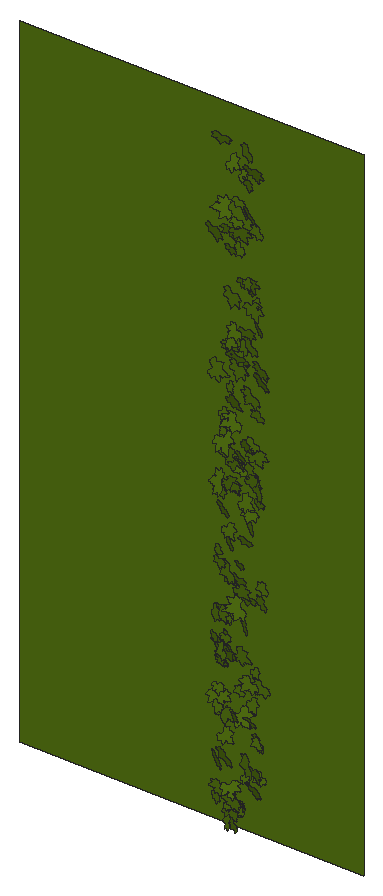
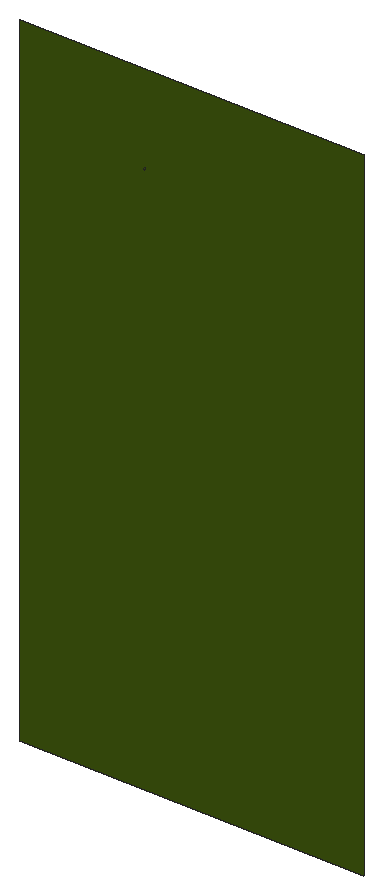
# SketchUp Ruby script. Lengths in inches.
U = 1.inch
M = Sketchup.active_model
def pt(a) = Geom::Point3d.new(a.map { |v| v * U })
def face(e, loops, mat)
  f = e.add_face(loops[0].map { |a| pt(a) })
  loops[1..].each { |l| e.add_face(l.map { |a| pt(a) }).erase! }
  f.material = f.back_material = mat if mat
  f
end
# faces: each face lists its corners as indices into pts; further lists are holes
def faces(e, pts, list, mat = nil) = list.each { |f| face(e, (f[0].is_a?(Array) ? f : [f]).map { |l| l.map { |i| pts[i] } }, mat) }
# xy, xz, yz: faces in a plane at the given z, y or x. An outline is a flat list of corners, or four numbers for a rectangle; further outlines are holes
def ring(l) = l.size == 4 ? [[l[0], l[1]], [l[2], l[1]], [l[2], l[3]], [l[0], l[3]]] : l.each_slice(2).to_a
def flat(e, list, mat, &to3) = list.each { |f| face(e, (f[0].is_a?(Array) ? f : [f]).map { |l| ring(l).map { |u, v| to3.(u, v) } }, mat) }
def xy(e, z, list, mat = nil) = flat(e, list, mat) { |x, y| [x, y, z] }
def xz(e, y, list, mat = nil) = flat(e, list, mat) { |x, z| [x, y, z] }
def yz(e, x, list, mat = nil) = flat(e, list, mat) { |y, z| [x, y, z] }
def lines(e, pts, list) = list.each { |a, b| e.add_line(pt(pts[a]), pt(pts[b])) }
# prism: a flat outline (further loops are holes) pulled along v
def prism(e, loops, v, mat = nil)
  f = face(e, loops, mat); d = Geom::Vector3d.new(v.map { |x| x * U })
  f.pushpull(f.normal.samedirection?(d) ? d.length : -d.length)
end
def box(e, o, s, mat = nil) = prism(e, [[o, [o[0] + s[0], o[1], o[2]], [o[0] + s[0], o[1] + s[1], o[2]], [o[0], o[1] + s[1], o[2]]]], [0, 0, s[2]], mat)
def at(x, y, z, deg = 0) = Geom::Transformation.translation(pt([x, y, z])) * Geom::Transformation.rotation(ORIGIN, Z_AXIS, deg.degrees)
def axes(o, x, y, z) = Geom::Transformation.new([*x, 0, *y, 0, *z, 0, *pt(o).to_a, 1])
def part(name) = M.definitions.add(name)
# library, detail: a bought-in or finely detailed component or shape, given as its bounding box
def library(name, o, s) = part(name).tap { |d| box(d.entities, o, s) }
def detail(e, o, s) = box(e.add_group.entities, o, s)
def put(e, d, t, mat = nil) = e.add_instance(d, t).tap { |i| i.material = mat if mat }
def group(e, t, mat = nil) = e.add_group.tap { |g| g.transformation = t; g.material = mat if mat }.entities
root = M.entities
M.materials.add("[Vegetation Blur 03]").color = [83, 114, 18]
c1 = part("ivy")
xy(c1.entities,0,[[0.782,0,0.786,0,0.787,0.005,0.789,0.009,0.821,0.072,0.875,0.147,1.001,0.272,1.073,0.331,1.137,0.363,1.178,0.379,1.223,0.384,1.272,0.383,1.311,0.374,1.36,0.355,1.399,0.334,1.491,0.285,1.541,0.244,1.583,0.199,1.617,0.15,1.64,0.128,1.662,0.115,1.717,0.105,1.745,0.093,1.784,0.054,1.819,0.057,1.854,0.064,1.882,0.075,1.896,0.074,1.91,0.071,1.937,0.063,1.964,0.053,1.99,0.038,2.016,0.015,2.034,0.002,2.04,0,2.038,0.003,2.036,0.007,2.033,0.038,2.036,0.068,2.045,0.1,2.055,0.116,2.064,0.123,2.077,0.129,2.088,0.129,2.106,0.132,2.118,0.13,2.179,0.132,2.207,0.133,2.225,0.133,2.242,0.138,2.22,0.162,2.207,0.186,2.206,0.213,2.212,0.236,2.228,0.262,2.247,0.274,2.298,0.283,2.355,0.294,2.37,0.296,2.376,0.295,2.377,0.3,2.377,0.303,2.385,0.329,2.411,0.37,2.426,0.392,2.449,0.407,2.511,0.426,2.561,0.444,2.619,0.466,2.589,0.469,2.561,0.476,2.501,0.5,2.449,0.516,2.424,0.523,2.401,0.535,2.377,0.556,2.372,0.568,2.36,0.575,2.268,0.586,2.225,0.592,2.207,0.599,2.194,0.61,2.143,0.65,2.13,0.664,2.122,0.682,2.123,0.7,2.13,0.719,2.148,0.75,2.17,0.781,2.195,0.807,2.221,0.828,2.284,0.874,2.291,0.88,2.288,0.887,2.276,0.9,2.267,0.916,2.265,0.933,2.273,0.967,2.292,1.002,2.313,1.03,2.334,1.054,2.348,1.067,2.358,1.074,2.363,1.076,2.362,1.081,2.35,1.094,2.347,1.11,2.35,1.143,2.359,1.18,2.385,1.254,2.415,1.324,2.448,1.393,2.45,1.4,2.446,1.398,2.44,1.394,2.427,1.383,2.402,1.36,2.376,1.339,2.345,1.324,2.305,1.309,2.282,1.303,2.273,1.306,2.245,1.294,2.212,1.287,2.187,1.291,2.163,1.301,2.142,1.316,2.134,1.327,2.124,1.325,2.09,1.292,2.053,1.259,2.014,1.234,1.973,1.215,1.954,1.21,1.931,1.208,1.909,1.212,1.893,1.22,1.879,1.233,1.872,1.248,1.867,1.281,1.864,1.319,1.821,1.258,1.773,1.197,1.726,1.141,1.698,1.121,1.679,1.116,1.666,1.117,1.647,1.122,1.632,1.129,1.62,1.141,1.617,1.154,1.617,1.219,1.621,1.254,1.623,1.268,1.623,1.281,1.618,1.314,1.606,1.346,1.603,1.375,1.607,1.403,1.603,1.467,1.599,1.499,1.605,1.525,1.614,1.552,1.629,1.577,1.635,1.589,1.629,1.587,1.618,1.582,1.596,1.566,1.581,1.556,1.568,1.552,1.557,1.55,1.545,1.553,1.531,1.562,1.522,1.572,1.504,1.591,1.486,1.611,1.474,1.631,1.457,1.666,1.455,1.684,1.457,1.698,1.452,1.715,1.444,1.728,1.424,1.754,1.419,1.772,1.423,1.786,1.434,1.819,1.444,1.848,1.446,1.855,1.44,1.861,1.43,1.867,1.386,1.904,1.349,1.948,1.326,1.973,1.31,1.995,1.288,2.048,1.284,2.153,1.287,2.254,1.284,2.255,1.282,2.253,1.278,2.247,1.274,2.237,1.266,2.216,1.226,2.125,1.208,2.076,1.184,2.033,1.155,1.984,1.135,1.942,1.111,1.899,1.083,1.861,1.053,1.85,1.059,1.83,1.061,1.809,1.056,1.79,1.049,1.767,1.04,1.749,1.018,1.733,0.994,1.726,0.942,1.734,0.95,1.6875,0.944,1.645,0.932,1.608,0.911,1.585,0.881,1.58,0.854,1.582,0.828,1.588,0.785,1.618,0.773,1.625,0.775,1.614,0.779,1.598,0.796,1.502,0.818,1.402,0.861,1.283,0.882,1.224,0.894,1.174,0.892,1.148,0.886,1.123,0.881,1.107,0.872,1.099,0.849,1.094,0.818,1.092,0.789,1.098,0.762,1.107,0.753,1.113,0.721,1.139,0.698,1.163,0.678,1.194,0.665,1.224,0.628,1.28,0.612,1.312,0.606,1.327,0.606,1.314,0.599,1.282,0.594,1.267,0.581,1.256,0.544,1.245,0.512,1.244,0.473,1.249,0.444,1.256,0.382,1.288,0.339,1.306,0.324,1.316,0.317,1.324,0.309,1.326,0.27,1.314,0.227,1.313,0.185,1.3125,0.152,1.317,0.122,1.328,0.092,1.345,0.073,1.353,0.079,1.338,0.092,1.308,0.117,1.249,0.13,1.215,0.139,1.164,0.147,1.148,0.157,1.136,0.163,1.122,0.174,1.086,0.177,1.067,0.182,1.054,0.186,1.043,0.191,1.038,0.211,1.028,0.237,1.005,0.25,0.974,0.253,0.96,0.25,0.944,0.242,0.914,0.243,0.906,0.249,0.902,0.26,0.894,0.289,0.88,0.307,0.873,0.322,0.862,0.364,0.799,0.403,0.738,0.431,0.709,0.439,0.691,0.441,0.678,0.4375,0.66,0.428,0.645,0.394,0.623,0.303,0.594,0.255,0.581,0.214,0.577,0.179,0.573,0.173,0.568,0.175,0.561,0.167,0.55,0.141,0.523,0.113,0.503,0.077,0.49,0.045,0.486,0.026,0.485,0.019,0.486,0.011,0.483,0,0.471,0.014,0.467,0.044,0.455,0.058,0.447,0.07,0.438,0.097,0.411,0.125,0.394,0.158,0.377,0.174,0.366,0.182,0.359,0.185,0.361,0.242,0.331,0.253,0.316,0.258,0.303,0.262,0.283,0.274,0.278,0.308,0.274,0.341,0.252,0.366,0.226,0.366,0.222,0.37,0.22,0.38,0.221,0.395,0.221,0.425,0.216,0.45,0.207,0.465,0.192,0.473,0.178,0.484,0.15,0.489,0.116,0.483,0.089,0.468,0.058,0.45,0.035,0.435,0.018,0.429,0.011,0.434,0.012,0.438,0.014,0.469,0.019,0.542,0.016,0.581,0.015,0.612,0.027,0.68,0.055,0.696,0.057,0.712,0.052,0.73,0.045,0.741,0.036,0.766,0.014]])
xz(root,174.5,[[114.28,101,138.74,147]],"[Vegetation Blur 03]")
put(root,c1,axes([128.08,173.7,139.49],[0.6079,-0.24736,0.08777],[0.11732,0.08596,-0.50313],[-0.11068,-1.26744,-0.05125]),"[Vegetation Blur 03]")
put(root,c1,axes([128.47,173.7,113.51],[0.3306,-0.20851,0.08999],[0.10594,-0.063,-0.2822],[-0.10584,-0.71438,-0.00138]),"[Vegetation Blur 03]")
put(root,c1,axes([128.72,173.7,113.4],[0.54219,-0.07189,-0.27942],[-0.3337,0.21166,-0.43986],[-0.08416,-1.30245,-0.05606]),"[Vegetation Blur 03]")
put(root,c1,axes([128.59,173.7,145.41],[0.46012,0.08661,-0.09796],[-0.12471,0.12465,-0.37281],[0.02504,-0.97055,-0.05662]),"[Vegetation Blur 03]")
put(root,c1,axes([128.5625,173.7,104.16],[0.58678,0.063,-0.19417],[-0.23912,0.05083,-0.47872],[0.01906,-1.30195,-0.02809]),"[Vegetation Blur 03]")
put(root,c1,axes([128.51,173.7,103.27],[0.34382,-0.15266,0.07768],[0.0934,-0.03785,-0.28706],[-0.07642,-0.73315,-0.00136]),"[Vegetation Blur 03]")
put(root,c1,axes([128.07,173.7,109.53],[0.59488,0.11123,0.16598],[0.20655,-0.0688,-0.48585],[0.04022,-1.29188,0.04016]),"[Vegetation Blur 03]")
put(root,c1,axes([128.54,173.7,106.05],[0.51362,-0.33546,-0.11294],[-0.11227,0.20752,-0.43703],[-0.18199,-1.07476,-0.04914]),"[Vegetation Blur 03]")
put(root,c1,axes([129.11,173.7,112.17],[0.24584,0.04332,-0.24097],[-0.29547,0.08344,-0.19842],[-0.01781,-0.78621,-0.03434]),"[Vegetation Blur 03]")
put(root,c1,axes([129.45,173.7,124.09],[0.21833,-0.37386,-0.44692],[-0.55988,0.15366,-0.2024],[-0.13932,-1.20335,0.113]),"[Vegetation Blur 03]")
put(root,c1,axes([129.2,173.7,106.26],[0.33588,0.02262,-0.39753],[-0.47681,0.26549,-0.26596],[-0.10014,-1.18823,-0.067]),"[Vegetation Blur 03]")
put(root,c1,axes([128.25,173.7,129.59],[0.09221,0.01276,0.54145],[0.66339,-0.02223,-0.07517],[-0.00985,-1.37816,0.00623]),"[Vegetation Blur 03]")
put(root,c1,axes([128.54,173.7,123.17],[0.25,-0.03131,0.17773],[0.21716,-0.03407,-0.2044],[-0.02234,-0.68141,0.00205]),"[Vegetation Blur 03]")
put(root,c1,axes([128.51,173.7,114.53],[0.13511,-0.04438,0.35866],[0.42367,-0.24214,-0.11102],[-0.11873,-0.91459,0.01199]),"[Vegetation Blur 03]")
put(root,c1,axes([128.75,173.7,109.24],[0.37736,-0.14693,-0.03133],[-0.04655,-0.08489,-0.31089],[-0.06637,-0.77592,0.03994]),"[Vegetation Blur 03]")
put(root,c1,axes([128.58,173.7,110.22],[0.36114,-0.04689,0.10699],[0.12628,-0.12494,-0.29255],[-0.0419,-0.78067,0.04039]),"[Vegetation Blur 03]")
put(root,c1,axes([128.98,173.7,112.5625],[0.39633,-0.13888,-0.234],[-0.27566,0.17367,-0.32719],[-0.1038,-0.99151,-0.02453]),"[Vegetation Blur 03]")
put(root,c1,axes([128.73,173.7,118.66],[0.10493,-0.03643,0.24088],[0.29195,-0.08918,-0.08683],[-0.04677,-0.63839,-0.00162]),"[Vegetation Blur 03]")
put(root,c1,axes([128.5625,173.7,122.63],[0.3534,-0.02851,0.14206],[0.17452,0.03242,-0.28817],[-0.00545,-0.81,-0.01653]),"[Vegetation Blur 03]")
put(root,c1,axes([128.7,173.7,118.42],[0.40755,-0.11351,-0.00014],[0.00098,0.01751,-0.33557],[-0.05515,-0.83847,-0.00699]),"[Vegetation Blur 03]")
put(root,c1,axes([129.01,173.7,122.03],[0.4235,-0.13743,-0.21645],[-0.24668,0.24247,-0.3457],[-0.1181,-0.99928,-0.05411]),"[Vegetation Blur 03]")
put(root,c1,axes([128.78,173.7,111.86],[0.26031,-0.0805,0.12545],[0.1556,0.01165,-0.21388],[-0.03078,-0.62197,-0.02024]),"[Vegetation Blur 03]")
put(root,c1,axes([128.65,173.7,115.28],[0.41549,-0.08208,0.11963],[0.15106,0.12998,-0.33542],[-0.01613,-0.89729,-0.05953]),"[Vegetation Blur 03]")
put(root,c1,axes([129.3125,173.7,113.2],[0.33509,-0.2609,-0.26753],[-0.3303,0.08476,-0.28857],[-0.12012,-0.96089,0.04719]),"[Vegetation Blur 03]")
put(root,c1,axes([129.64,173.7,113.78],[0.07952,-0.02515,-0.25316],[-0.29832,0.17612,-0.06516],[-0.08589,-0.63499,-0.00805]),"[Vegetation Blur 03]")
put(root,c1,axes([129.88,173.7,141.66],[0.17867,-0.14742,-0.47769],[-0.58909,-0.10072,-0.14187],[0.02629,-1.25528,0.06748]),"[Vegetation Blur 03]")
put(root,c1,axes([130.06,173.7,125.72],[0.10377,0.02186,-0.53621],[-0.65451,0.12482,-0.08356],[-0.05827,-1.36305,-0.01625]),"[Vegetation Blur 03]")
put(root,c1,axes([129.85,173.7,114.94],[0.04974,-0.00028,-0.27725],[-0.32677,0.19308,-0.03908],[-0.09286,-0.67961,-0.01099]),"[Vegetation Blur 03]")
put(root,c1,axes([129.9375,173.7,115.46],[0.08632,-0.07212,-0.36138],[-0.4424,0.06914,-0.07256],[-0.03977,-0.92577,0.02273]),"[Vegetation Blur 03]")
put(root,c1,axes([129.62,173.7,118.4375],[0.39881,-0.16855,-0.40776],[-0.49292,0.16963,-0.33214],[-0.11562,-1.30452,0.00949]),"[Vegetation Blur 03]")
put(root,c1,axes([128.95,173.7,127.48],[0.21376,-0.00368,0.2636],[0.3197,-0.11113,-0.17293],[-0.04601,-0.78924,0.02312]),"[Vegetation Blur 03]")
put(root,c1,axes([129.32,173.7,127.12],[0.30532,-0.22387,-0.07925],[-0.10993,-0.04866,-0.26046],[-0.09582,-0.65751,0.04626]),"[Vegetation Blur 03]")
put(root,c1,axes([129.85,173.7,102.12],[0.10497,-0.16799,-0.28426],[-0.34085,0.17977,-0.10055],[-0.10859,-0.72666,0.04084]),"[Vegetation Blur 03]")
put(root,c1,axes([129.12,173.7,113.5625],[0.3425,-0.04443,0.04433],[0.05384,-0.01893,-0.28004],[-0.02276,-0.71335,0.00467]),"[Vegetation Blur 03]")
put(root,c1,axes([128.69,173.7,109.03],[0.66487,-0.12258,0.05657],[0.06821,-0.03171,-0.54475],[-0.06083,-1.37523,0.00752]),"[Vegetation Blur 03]")
put(root,c1,axes([129.74,173.7,119.85],[0.19183,-0.05588,-0.2698],[-0.31224,0.23474,-0.15552],[-0.11192,-0.75067,-0.02855]),"[Vegetation Blur 03]")
put(root,c1,axes([128.74,173.7,114.98],[0.40007,-0.13518,0.27607],[0.33165,-0.13835,-0.33079],[-0.0935,-1.06919,0.0079]),"[Vegetation Blur 03]")
put(root,c1,axes([128.82,173.7,106.75],[0.24435,0.09355,0.35761],[0.44053,-0.04867,-0.19849],[0.00137,-1.03125,0.04181]),"[Vegetation Blur 03]")
put(root,c1,axes([128.52,173.7,125.74],[0.49312,0.07516,0.37451],[0.45503,-0.28887,-0.38996],[-0.06962,-1.3557,0.10386]),"[Vegetation Blur 03]")
put(root,c1,axes([129.34,173.7,102.54],[0.09713,0.02395,0.23937],[0.28996,-0.10667,-0.07669],[-0.04564,-0.62678,0.0222]),"[Vegetation Blur 03]")
put(root,c1,axes([129.15,173.7,132.24],[0.48068,0.01776,0.03152],[0.03794,0.06838,-0.39147],[0.01124,-0.98997,-0.02647]),"[Vegetation Blur 03]")
put(root,c1,axes([129.13,173.7,102.32],[0.46585,0.02288,0.14137],[0.17091,0.11775,-0.37813],[0.0303,-1.01595,-0.04064]),"[Vegetation Blur 03]")
put(root,c1,axes([129.68,173.7,113.05],[0.36602,-0.17334,-0.17958],[-0.2031,0.19186,-0.30487],[-0.11941,-0.85763,-0.0319]),"[Vegetation Blur 03]")
put(root,c1,axes([129.08,173.7,139.67],[0.63593,0.00439,0.02808],[0.0337,0.19557,-0.51321],[0.00724,-1.29586,-0.07736]),"[Vegetation Blur 03]")
put(root,c1,axes([129.51,173.7,138.55],[0.37054,-0.08411,-0.02834],[-0.02969,0.09383,-0.30232],[-0.04467,-0.76008,-0.03419]),"[Vegetation Blur 03]")
put(root,c1,axes([129.06,173.7,103.84],[0.46596,0.12424,0.22352],[0.28037,-0.18097,-0.37349],[0.00652,-1.09739,0.0869]),"[Vegetation Blur 03]")
put(root,c1,axes([129.39,173.7,117.06],[0.25004,-0.05522,0.19659],[0.24228,0.07618,-0.20189],[0.00655,-0.71038,-0.03693]),"[Vegetation Blur 03]")
put(root,c1,axes([129.89,173.7,103.81],[0.43018,0.03461,-0.33433],[-0.40999,0.03807,-0.35076],[-0.00059,-1.2218,-0.0204]),"[Vegetation Blur 03]")
put(root,c1,axes([129.32,173.7,112.03],[0.13975,-0.17275,0.35559],[0.44281,0.11446,-0.10717],[0.0284,-0.9346,-0.07885]),"[Vegetation Blur 03]")
put(root,c1,axes([129.14,173.7,120.2],[0.35229,-0.00554,0.29733],[0.36145,-0.12544,-0.28562],[-0.04568,-1.0353,0.03302]),"[Vegetation Blur 03]")
put(root,c1,axes([130.07,173.7,128.11],[0.3559,-0.06669,-0.38571],[-0.47242,-0.14005,-0.28653],[0.03508,-1.20938,0.05445]),"[Vegetation Blur 03]")
put(root,c1,axes([129.41,173.7,103.72],[0.62299,-0.15418,-0.12642],[-0.15294,0.05244,-0.51207],[-0.07884,-1.31998,-0.00558]),"[Vegetation Blur 03]")
put(root,c1,axes([129.38,173.7,131.97],[0.08788,0.15958,0.41108],[0.50211,-0.20702,-0.05886],[-0.08717,-1.03158,0.0754]),"[Vegetation Blur 03]")
put(root,c1,axes([128.98,173.7,123.21],[0.49372,-0.08066,0.3359],[0.41334,0.06825,-0.4021],[-0.00879,-1.32093,-0.04129]),"[Vegetation Blur 03]")
put(root,c1,axes([129.875,173.7,102.14],[0.34936,-0.1754,-0.17065],[-0.20005,0.12722,-0.29335],[-0.10473,-0.82812,-0.00892]),"[Vegetation Blur 03]")
put(root,c1,axes([129.7,173.7,123.82],[0.46927,-0.11869,-0.14311],[-0.17217,0.07416,-0.3857],[-0.06659,-1.02821,-0.0113]),"[Vegetation Blur 03]")
put(root,c1,axes([129.56,173.7,129.45],[0.20111,-0.0492,0.23305],[0.27447,-0.17313,-0.16352],[-0.08231,-0.69755,0.02415]),"[Vegetation Blur 03]")
put(root,c1,axes([129.61,173.7,131.9375],[0.61818,0.02753,-0.20694],[-0.25253,0.20999,-0.49806],[-0.0265,-1.35881,-0.08116]),"[Vegetation Blur 03]")
put(root,c1,axes([129.48,173.7,143.34],[0.1221,0.15901,0.36769],[0.45566,-0.11863,-0.09271],[-0.03634,-0.95319,0.07288]),"[Vegetation Blur 03]")
put(root,c1,axes([129.77,173.7,103.77],[0.53938,-0.11783,-0.24861],[-0.28048,0.34993,-0.43141],[-0.13192,-1.22575,-0.09926]),"[Vegetation Blur 03]")
put(root,c1,axes([129.49,173.7,109.0625],[0.49941,-0.26714,0.04177],[0.06827,0.12648,-0.4165],[-0.1217,-1.02529,-0.06226]),"[Vegetation Blur 03]")
put(root,c1,axes([130.68,173.7,141.38],[0.10747,0.09693,-0.42949],[-0.50045,0.37307,-0.07017],[-0.16944,-1.0404,-0.06517]),"[Vegetation Blur 03]")
put(root,c1,axes([129.47,173.7,135.95],[0.66254,-0.24066,-0.04091],[-0.05165,-0.00895,-0.54898],[-0.11628,-1.36725,0.01079]),"[Vegetation Blur 03]")
put(root,c1,axes([130.08,173.7,133.8],[0.41213,-0.1677,-0.21359],[-0.27008,-0.08234,-0.33694],[-0.04682,-1.00125,0.06348]),"[Vegetation Blur 03]")
put(root,c1,axes([130.57,173.7,116.5],[0.32603,-0.13943,-0.47145],[-0.58131,-0.12239,-0.26207],[0.01889,-1.35947,0.07195]),"[Vegetation Blur 03]")
put(root,c1,axes([130.01,173.7,140.4],[0.32282,0.01218,-0.05233],[-0.06347,-0.05325,-0.26277],[0.01083,-0.67519,0.01978]),"[Vegetation Blur 03]")
put(root,c1,axes([129.6,173.7,124.54],[0.35919,-0.07581,0.24051],[0.29623,0.02355,-0.29351],[-0.02119,-0.9558,-0.02631]),"[Vegetation Blur 03]")
put(root,c1,axes([130.18,173.7,141.8],[0.32239,-0.01176,-0.10948],[-0.13423,-0.01041,-0.2631],[-0.00333,-0.71849,0.00561]),"[Vegetation Blur 03]")
put(root,c1,axes([130.7,173.7,103.01],[0.06839,0.01536,-0.24268],[-0.29667,-0.04173,-0.0561],[0.02144,-0.62648,-0.00221]),"[Vegetation Blur 03]")
put(root,c1,axes([130.6,173.7,110.71],[0.15181,-0.00524,-0.23084],[-0.28286,-0.00517,-0.12389],[0.00101,-0.66057,0.0028]),"[Vegetation Blur 03]")
put(root,c1,axes([129.49,173.7,128.62],[0.38193,-0.25872,0.35613],[0.44798,0.02235,-0.31745],[-0.07443,-1.19311,-0.08317]),"[Vegetation Blur 03]")
put(root,c1,axes([130.93,173.7,114.9],[0.06026,0.01776,-0.40154],[-0.46093,0.35917,-0.04358],[-0.17229,-0.95467,-0.02387]),"[Vegetation Blur 03]")
put(root,c1,axes([130.36,173.7,125.6],[0.28037,-0.06157,-0.15463],[-0.18018,0.15229,-0.22714],[-0.06579,-0.67947,-0.0369]),"[Vegetation Blur 03]")
put(root,c1,axes([129.96,173.7,117.7],[0.47998,-0.11829,-0.01678],[-0.01365,0.11877,-0.39191],[-0.0595,-0.98146,-0.0454]),"[Vegetation Blur 03]")
put(root,c1,axes([130.1875,173.7,118.55],[0.3065,-0.10801,0.00878],[0.01921,0.10156,-0.25024],[-0.05001,-0.62289,-0.04232]),"[Vegetation Blur 03]")
put(root,c1,axes([129.91,173.7,131.42],[0.63233,-0.20373,-0.05495],[-0.06893,-0.01048,-0.5222],[-0.0979,-1.30853,0.01274]),"[Vegetation Blur 03]")
put(root,c1,axes([129.64,173.7,139.53],[0.56255,-0.01811,0.20546],[0.25121,0.13405,-0.45628],[0.01862,-1.26114,-0.05145]),"[Vegetation Blur 03]")
put(root,c1,axes([130.77,173.7,124.98],[0.19807,-0.04882,-0.25327],[-0.31096,-0.06252,-0.16009],[0.01294,-0.755,0.02963]),"[Vegetation Blur 03]")
put(root,c1,axes([130.14,173.7,125.22],[0.42582,-0.25778,-0.01572],[0.00049,0.14225,-0.35818],[-0.12674,-0.86554,-0.05419]),"[Vegetation Blur 03]")
put(root,c1,axes([130.65,173.7,120.24],[0.26692,0.10027,-0.19485],[-0.24358,0.09015,-0.21495],[0.00657,-0.73139,-0.05321]),"[Vegetation Blur 03]")
put(root,c1,axes([130.39,173.7,139.04],[0.38208,-0.19358,-0.10183],[-0.13229,-0.03969,-0.31874],[-0.08317,-0.82615,0.03917]),"[Vegetation Blur 03]")
put(root,c1,axes([129.7,173.7,108.34],[0.39393,0.1891,0.39235],[0.48905,-0.10099,-0.3194],[0.01969,-1.27498,0.08349]),"[Vegetation Blur 03]")
put(root,c1,axes([130.13,173.7,130.7],[0.23197,-0.0436,0.29061],[0.3566,0.00644,-0.18945],[-0.00894,-0.8745,-0.01588]),"[Vegetation Blur 03]")
put(root,c1,axes([131.08,173.7,106.44],[0.28462,-0.17247,-0.45638],[-0.54186,0.28495,-0.24203],[-0.16158,-1.25936,0.00774]),"[Vegetation Blur 03]")
put(root,c1,axes([129.94,173.7,116.58],[0.39343,-0.07208,0.30532],[0.37571,0.06003,-0.32024],[-0.0052,-1.11557,-0.03696]),"[Vegetation Blur 03]")
put(root,c1,axes([130.43,173.7,142.95],[0.0888,0.09674,0.25308],[0.31076,-0.1168,-0.0656],[-0.0424,-0.6534,0.0492]),"[Vegetation Blur 03]")
put(root,c1,axes([130.86,173.7,132.92],[0.29115,-0.21346,-0.2217],[-0.27097,0.0878,-0.25032],[-0.10549,-0.81469,0.03111]),"[Vegetation Blur 03]")
put(root,c1,axes([131.38,173.7,125.1],[0.14596,0.116,-0.44941],[-0.55223,-0.05004,-0.12149],[0.03805,-1.17121,-0.03932]),"[Vegetation Blur 03]")
put(root,c1,axes([130.11,173.7,112.21],[0.18573,-0.07263,0.44986],[0.55141,-0.04477,-0.15278],[-0.03192,-1.19609,-0.0216]),"[Vegetation Blur 03]")
put(root,c1,axes([130.61,173.7,116.51],[0.38415,0.08832,-0.09325],[-0.11924,0.10565,-0.31143],[0.02608,-0.81794,-0.0503]),"[Vegetation Blur 03]")
put(root,c1,axes([130.87,173.7,141.38],[0.42548,-0.09437,-0.33716],[-0.38139,0.39508,-0.33797],[-0.16527,-1.15464,-0.08808]),"[Vegetation Blur 03]")
put(root,c1,axes([130.9375,173.7,145.45],[0.35368,-0.15187,-0.29343],[-0.34945,0.17479,-0.29479],[-0.11221,-1.02299,-0.00681]),"[Vegetation Blur 03]")
put(root,c1,axes([131.05,173.7,108.8],[0.21856,0.08137,-0.22546],[-0.27868,0.10188,-0.17416],[-0.01478,-0.71768,-0.05028]),"[Vegetation Blur 03]")
put(root,c1,axes([130.53,173.7,104.72],[0.17985,0.03398,0.21034],[0.25744,-0.07475,-0.14472],[-0.02044,-0.64238,0.02797]),"[Vegetation Blur 03]")
put(root,c1,axes([131.03,173.7,133.11],[0.38374,-0.03816,-0.34105],[-0.41282,0.15382,-0.31209],[-0.06752,-1.15732,-0.03024]),"[Vegetation Blur 03]")
put(root,c1,axes([131.4,173.7,121.25],[0.07886,-0.02245,-0.3122],[-0.36365,0.24601,-0.06396],[-0.11923,-0.76517,-0.0114]),"[Vegetation Blur 03]")
put(root,c1,axes([130.33,173.7,121.98],[0.16307,0.08475,0.41488],[0.5096,-0.07153,-0.13111],[-0.02064,-1.09626,0.04063]),"[Vegetation Blur 03]")
put(root,c1,axes([130.96,173.7,111.56],[0.42678,-0.01115,-0.26433],[-0.32354,-0.0687,-0.34749],[0.01587,-1.10035,0.02437]),"[Vegetation Blur 03]")
put(root,c1,axes([130.35,173.7,133.48],[0.51847,-0.08238,0.09913],[0.12469,0.09368,-0.42215],[-0.02842,-1.09178,-0.0437]),"[Vegetation Blur 03]")
put(root,c1,axes([130.16,173.7,136.53],[0.5764,-0.04158,0.19028],[0.23362,0.17732,-0.46527],[0.01378,-1.26714,-0.07135]),"[Vegetation Blur 03]")
put(root,c1,axes([131.01,173.7,136.41],[0.29856,-0.10941,-0.11062],[-0.12269,0.1536,-0.24445],[-0.0784,-0.65702,-0.03873]),"[Vegetation Blur 03]")
put(root,c1,axes([130.96,173.7,130.02],[0.54012,-0.12372,-0.29412],[-0.3556,0.12595,-0.44329],[-0.0839,-1.33021,-0.01462]),"[Vegetation Blur 03]")
put(root,c1,axes([130.8,173.7,122.15],[0.44019,0.01869,-0.05575],[-0.06711,-0.08998,-0.3577],[0.01564,-0.91223,0.03414]),"[Vegetation Blur 03]")
put(root,c1,axes([130.57,173.7,126.07],[0.25746,-0.20708,0.31713],[0.39391,-0.05224,-0.21837],[-0.07715,-0.95777,-0.05666]),"[Vegetation Blur 03]")
put(root,c1,axes([130.7,173.7,143.22],[0.42985,-0.21428,0.06487],[0.08397,0.02008,-0.36019],[-0.10055,-0.89931,-0.0235]),"[Vegetation Blur 03]")
put(root,c1,axes([130.72,173.7,136.5],[0.26598,-0.07146,0.22657],[0.27016,-0.13937,-0.21816],[-0.07275,-0.7788,0.01825]),"[Vegetation Blur 03]")
put(root,c1,axes([131.25,173.7,126.82],[0.32974,-0.02071,-0.22461],[-0.27537,-0.01528,-0.26905],[-0.00296,-0.88368,0.00992]),"[Vegetation Blur 03]")
put(root,c1,axes([131.83,173.7,128.67],[0.16409,0.0678,-0.30247],[-0.37206,0.03564,-0.13319],[-0.00256,-0.83328,-0.0303]),"[Vegetation Blur 03]")
put(root,c1,axes([130.82,173.7,123.74],[0.26787,-0.06927,0.33281],[0.40897,0.07748,-0.21671],[0.01312,-1.00101,-0.0398]),"[Vegetation Blur 03]")
put(root,c1,axes([130.68,173.7,143.96],[0.62307,-0.149,0.09151],[0.12235,0.19755,-0.50432],[-0.05332,-1.28769,-0.08796]),"[Vegetation Blur 03]")
put(root,c1,axes([131.74,173.7,107.95],[0.28434,-0.07307,-0.35446],[-0.41994,0.239,-0.23213],[-0.11635,-1.04116,-0.02841]),"[Vegetation Blur 03]")
put(root,c1,axes([131.84,173.7,140.49],[0.19509,-0.01615,-0.32843],[-0.40182,0.04546,-0.15934],[-0.0233,-0.91916,-0.00211]),"[Vegetation Blur 03]")
put(root,c1,axes([130.89,173.7,104.75],[0.57489,-0.26657,0.03866],[0.06843,0.18847,-0.47339],[-0.11976,-1.17196,-0.08492]),"[Vegetation Blur 03]")
put(root,c1,axes([131.79,173.7,124.49],[0.3874,-0.28987,-0.42046],[-0.49062,0.32448,-0.33628],[-0.21109,-1.28615,0.00992]),"[Vegetation Blur 03]")
put(root,c1,axes([130.95,173.7,109.6875],[0.31135,-0.03304,0.2876],[0.34314,-0.19604,-0.25097],[-0.08184,-0.94759,0.04189]),"[Vegetation Blur 03]")
put(root,c1,axes([131.82,173.7,107.82],[0.20749,-0.03484,-0.23563],[-0.28917,-0.01288,-0.16931],[-0.00479,-0.73151,0.0142]),"[Vegetation Blur 03]")
put(root,c1,axes([130.71,173.7,135.15],[0.58643,-0.10608,0.2337],[0.28408,-0.0778,-0.48036],[-0.06289,-1.34069,0.00938]),"[Vegetation Blur 03]")
put(root,c1,axes([130.83,173.7,125.65],[0.54429,0.0275,0.19656],[0.23996,0.06284,-0.44397],[0.02457,-1.22318,-0.01839]),"[Vegetation Blur 03]")
put(root,c1,axes([131.27,173.7,111.82],[0.22624,-0.03067,0.2044],[0.24637,-0.10398,-0.18409],[-0.04741,-0.6867,0.01875]),"[Vegetation Blur 03]")
put(root,c1,axes([132.18,173.7,116.83],[0.12874,0.00958,-0.35889],[-0.43298,0.16781,-0.10275],[-0.07698,-0.92784,-0.02229]),"[Vegetation Blur 03]")
put(root,c1,axes([131.68,173.7,131.04],[0.44147,-0.0788,-0.2903],[-0.33877,0.28169,-0.35517],[-0.11502,-1.13213,-0.06817]),"[Vegetation Blur 03]")
put(root,c1,axes([131.87,173.7,105.77],[0.29889,-0.0519,-0.2268],[-0.27904,-0.05258,-0.24304],[-0.001,-0.83818,0.02929]),"[Vegetation Blur 03]")
put(root,c1,axes([131.45,173.7,135.43],[0.18943,-0.02258,0.18927],[0.22327,-0.15119,-0.15168],[-0.06367,-0.59736,0.03124]),"[Vegetation Blur 03]")
put(root,c1,axes([131.11,173.7,105.71],[0.48095,-0.24511,0.14889],[0.18901,0.01686,-0.4023],[-0.10837,-1.05836,-0.04089]),"[Vegetation Blur 03]")
put(root,c1,axes([131.6,173.7,122.97],[0.32248,-0.05987,-0.04087],[-0.04757,0.05862,-0.26354],[-0.03303,-0.669,-0.01944]),"[Vegetation Blur 03]")
put(root,c1,axes([131.66,173.7,134.23],[0.34481,-0.20074,-0.10306],[-0.10927,0.15385,-0.29065],[-0.11628,-0.7398,-0.03248]),"[Vegetation Blur 03]")
put(root,c1,axes([131.7,173.7,111.59],[0.47072,-0.03676,-0.23219],[-0.28418,0.02801,-0.38445],[-0.02233,-1.13149,-0.00197]),"[Vegetation Blur 03]")
put(root,c1,axes([132.27,173.7,117.86],[0.16539,-0.02327,-0.29289],[-0.35869,0.02592,-0.13523],[-0.01618,-0.81273,0.00407]),"[Vegetation Blur 03]")
put(root,c1,axes([131.53,173.7,131.81],[0.56634,-0.19077,-0.13861],[-0.15859,0.16167,-0.4666],[-0.11086,-1.2059,-0.04063]),"[Vegetation Blur 03]")
